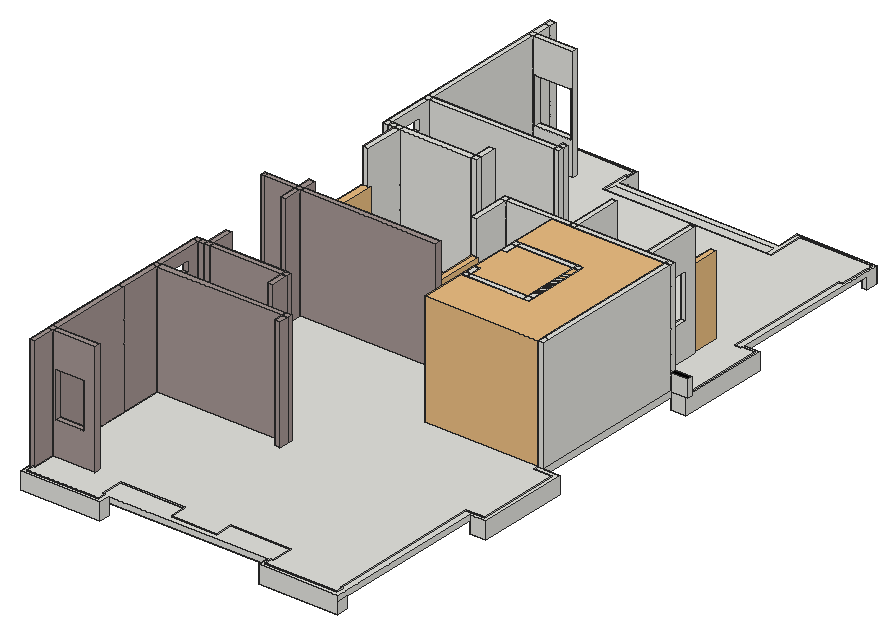
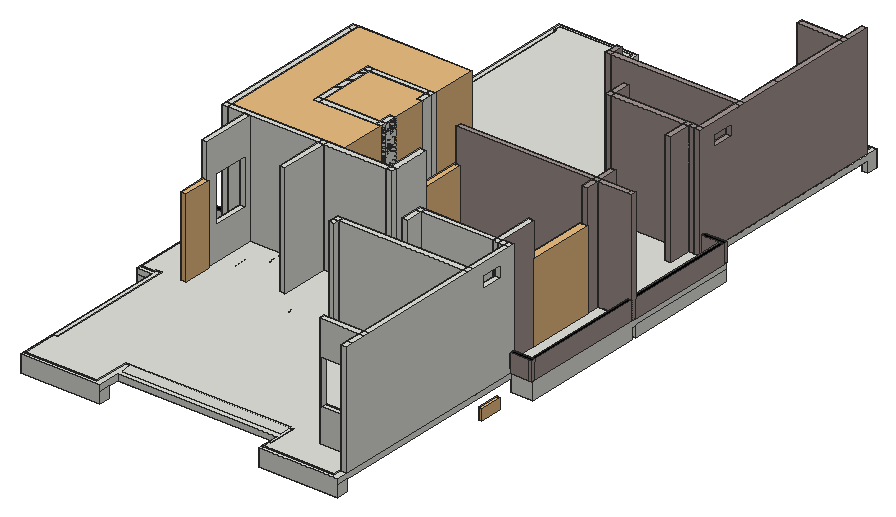
# SketchUp Ruby script. Lengths in inches.
U = 1.inch
M = Sketchup.active_model
def pt(a) = Geom::Point3d.new(a.map { |v| v * U })
def face(e, loops, mat)
  f = e.add_face(loops[0].map { |a| pt(a) })
  loops[1..].each { |l| e.add_face(l.map { |a| pt(a) }).erase! }
  f.material = f.back_material = mat if mat
  f
end
# faces: each face lists its corners as indices into pts; further lists are holes
def faces(e, pts, list, mat = nil) = list.each { |f| face(e, (f[0].is_a?(Array) ? f : [f]).map { |l| l.map { |i| pts[i] } }, mat) }
# xy, xz, yz: faces in a plane at the given z, y or x. An outline is a flat list of corners, or four numbers for a rectangle; further outlines are holes
def ring(l) = l.size == 4 ? [[l[0], l[1]], [l[2], l[1]], [l[2], l[3]], [l[0], l[3]]] : l.each_slice(2).to_a
def flat(e, list, mat, &to3) = list.each { |f| face(e, (f[0].is_a?(Array) ? f : [f]).map { |l| ring(l).map { |u, v| to3.(u, v) } }, mat) }
def xy(e, z, list, mat = nil) = flat(e, list, mat) { |x, y| [x, y, z] }
def xz(e, y, list, mat = nil) = flat(e, list, mat) { |x, z| [x, y, z] }
def yz(e, x, list, mat = nil) = flat(e, list, mat) { |y, z| [x, y, z] }
def lines(e, pts, list) = list.each { |a, b| e.add_line(pt(pts[a]), pt(pts[b])) }
# prism: a flat outline (further loops are holes) pulled along v
def prism(e, loops, v, mat = nil)
  f = face(e, loops, mat); d = Geom::Vector3d.new(v.map { |x| x * U })
  f.pushpull(f.normal.samedirection?(d) ? d.length : -d.length)
end
def box(e, o, s, mat = nil) = prism(e, [[o, [o[0] + s[0], o[1], o[2]], [o[0] + s[0], o[1] + s[1], o[2]], [o[0], o[1] + s[1], o[2]]]], [0, 0, s[2]], mat)
def at(x, y, z, deg = 0) = Geom::Transformation.translation(pt([x, y, z])) * Geom::Transformation.rotation(ORIGIN, Z_AXIS, deg.degrees)
def axes(o, x, y, z) = Geom::Transformation.new([*x, 0, *y, 0, *z, 0, *pt(o).to_a, 1])
def part(name) = M.definitions.add(name)
# library, detail: a bought-in or finely detailed component or shape, given as its bounding box
def library(name, o, s) = part(name).tap { |d| box(d.entities, o, s) }
def detail(e, o, s) = box(e.add_group.entities, o, s)
def put(e, d, t, mat = nil) = e.add_instance(d, t).tap { |i| i.material = mat if mat }
def group(e, t, mat = nil) = e.add_group.tap { |g| g.transformation = t; g.material = mat if mat }.entities
root = M.entities
M.materials.add("M09_Shadow_Night").color = [0, 0, 0]
M.materials.add("Marble_06_1K").color = [165, 150, 147]
c1 = part("Group\#53")
xy(c1.entities,0,[[-66,-66,-60,-60],[-60,-66,0,-60],[0,-66,6,-60],[-66,-60,-60,-48.73],[0,-60,6,0],
  [-66,-12.73,-60,0],[-66,0,-60,6],[-60,0,0,6],[0,0,6,6]])
xy(c1.entities,120,[[-66,-66,-60,-60],[-60,-66,0,-60],[0,-66,6,-60],[-66,-60,-60,-48.73],[0,-60,6,0],
  [-66,-12.73,-60,0],[-66,0,-60,6],[-60,0,0,6],[0,0,6,6]])
xz(c1.entities,-66,[[-66,0,-60,120],[-60,0,0,120],[0,0,6,120]])
xz(c1.entities,-60,[[-66,0,-60,120],[-60,0,0,120],[0,0,6,120]])
xz(c1.entities,-48.73,[[-66,0,-60,120]])
xz(c1.entities,-12.73,[[-66,0,-60,120]])
xz(c1.entities,0,[[-66,0,-60,120],[-60,0,0,120],[0,0,6,120]])
xz(c1.entities,6,[[-66,0,-60,120],[-60,0,0,120],[0,0,6,120]])
yz(c1.entities,-66,[[-66,0,-60,120],[-60,0,-48.73,120],[-12.73,0,0,120],[0,0,6,120]])
yz(c1.entities,-60,[[-66,0,-60,120],[-60,0,-48.73,120],[-12.73,0,0,120],[0,0,6,120]])
yz(c1.entities,0,[[-66,0,-60,120],[-60,0,0,120],[0,0,6,120]])
yz(c1.entities,6,[[-66,0,-60,120],[-60,0,0,120],[0,0,6,120]])
c2 = library("Return staircase",[0,-11.89,0],[120,168,120])
c3 = part("Group\#84")
xy(c3.entities,0,[[[-2,-32,-2,-24,0.04,-24,0.04,0,0,0,0,198,-6,198,-6,196,-25.9,196,-25.9,312.57,0,312.57,0,318.21,-25.9,318.21,-25.9,446,-6,446,-6,444,0,444,0,675.78,72,673.93,76,673.93,76,665.93,74,665.93,74,636,252.4,636,252.4,673.93,328.4,673.93,328.4,636,324.4,636,324.4,498.14,330.4,498.14,330.4,499.84,344.35,499.84,344.35,411,324.4,411,324.4,231,344.35,231,344.35,142,324.4,142,324.4,0,324.58,0,324.58,-24,326.4,-24,326.4,-32,250.4,-32,250.4,-24,252.4,-24,252.4,0,188.4,0,188.4,-18,140,-18,140,0,72,0,72,-24,74,-24,74,-32],[210.4,291,270.4,351]]])
xy(c3.entities,1,[[[-2,-32,74,-32,74,-24,72,-24,72,0,140,0,140,-18,188.4,-18,188.4,0,252.4,0,252.4,-24,250.4,-24,250.4,-32,326.4,-32,326.4,-24,324.58,-24,324.58,0,324.4,0,324.4,142,344.35,142,344.35,231,324.4,231,324.4,411,344.35,411,344.35,499.84,330.4,499.84,330.4,498.14,324.4,498.14,324.4,636,328.4,636,328.4,673.93,252.4,673.93,252.4,636,74,636,74,665.93,76,665.93,76,673.93,72,673.93,0,675.78,0,444,-6,444,-6,446,-25.9,446,-25.9,318.21,0,318.21,0,312.57,-25.9,312.57,-25.9,196,-6,196,-6,198,0,198,0,0,0.04,0,0.04,-24,-2,-24],[210.4,291,270.4,351]]])
xz(c3.entities,-32,[[-2,0,74,1],[250.4,0,326.4,1]])
xz(c3.entities,-24,[[-2,0,0.04,1],[72,0,74,1],[250.4,0,252.4,1],[324.58,0,326.4,1]])
xz(c3.entities,-18,[[140,0,188.4,1]])
xz(c3.entities,0,[[0,0,0.04,1],[72,0,140,1],[188.4,0,252.4,1],[324.4,0,324.58,1]])
xz(c3.entities,142,[[324.4,0,344.35,1]])
xz(c3.entities,196,[[-25.9,0,-6,1]])
xz(c3.entities,198,[[-6,0,0,1]])
xz(c3.entities,231,[[324.4,0,344.35,1]])
xz(c3.entities,291,[[210.4,0,270.4,1]])
xz(c3.entities,312.57,[[-25.9,0,0,1]])
xz(c3.entities,318.21,[[-25.9,0,0,1]])
xz(c3.entities,351,[[210.4,0,270.4,1]])
xz(c3.entities,411,[[324.4,0,344.35,1]])
xz(c3.entities,444,[[-6,0,0,1]])
xz(c3.entities,446,[[-25.9,0,-6,1]])
xz(c3.entities,498.14,[[324.4,0,330.4,1]])
xz(c3.entities,499.84,[[330.4,0,344.35,1]])
xz(c3.entities,636,[[74,0,252.4,1],[324.4,0,328.4,1]])
xz(c3.entities,665.93,[[74,0,76,1]])
xz(c3.entities,673.93,[[72,0,76,1],[252.4,0,328.4,1]])
yz(c3.entities,-25.9,[[196,0,312.57,1],[318.21,0,446,1]])
yz(c3.entities,-6,[[196,0,198,1],[444,0,446,1]])
yz(c3.entities,-2,[[-32,0,-24,1]])
yz(c3.entities,0,[[0,0,198,1],[312.57,0,318.21,1],[444,0,636,1],[636,0,637.85,1],[637.85,0,675.78,1]])
yz(c3.entities,0.04,[[-24,0,0,1]])
yz(c3.entities,72,[[-24,0,0,1]])
yz(c3.entities,74,[[-32,0,-24,1],[636,0,665.93,1]])
yz(c3.entities,76,[[665.93,0,673.93,1]])
yz(c3.entities,140,[[-18,0,0,1]])
yz(c3.entities,188.4,[[-18,0,0,1]])
yz(c3.entities,210.4,[[291,0,351,1]])
yz(c3.entities,250.4,[[-32,0,-24,1]])
yz(c3.entities,252.4,[[-24,0,0,1],[636,0,673.93,1]])
yz(c3.entities,270.4,[[291,0,351,1]])
yz(c3.entities,324.4,[[0,0,142,1],[231,0,411,1],[498.14,0,636,1]])
yz(c3.entities,324.58,[[-24,0,0,1]])
yz(c3.entities,326.4,[[-32,0,-24,1]])
yz(c3.entities,328.4,[[636,0,673.93,1]])
yz(c3.entities,330.4,[[498.14,0,499.84,1]])
yz(c3.entities,344.35,[[142,0,231,1],[411,0,499.84,1]])
p = [[77.67,648,0],[77.67,636,1],[246.4,636,1],[246.4,648,0],[72,673.93,0],[0,675.78,0],
  [0,675.78,1],[72,673.93,1],[70,636,0],[74,636,0],[42,642,0],[13.06,642,0],
  [13.06,673.93,0],[42,673.93,0]]
faces(c3.entities,p,[[0,1,2,3],[4,5,6,7]])
lines(c3.entities,p,[[8,9],[10,11],[12,13]])
c4 = library("TREE-26",[-60.96,-72.91,0],[121.92,134.74,0.01])
c5 = library("HYHHYHYHYHYHY",[-2.09,-4.54,0],[4.18,9.08,0.01])
c6 = library("Group\#51",[0,0,0],[6.9375,42,86.5])
c7 = part("feeeeeeeeee")
p = [[-2.68,3.51,0],[-2.68,3.16,0],[-2.92,3.16,0],[-2.92,3.07,0],[-3.56,3.07,0],[-3.56,3.51,0],
  [-2.68,-3.51,0],[-2.68,-3.16,0],[-2.92,-3.16,0],[-2.92,-3.07,0],[-3.56,-3.07,0],[-3.56,-3.51,0],
  [3.56,3.16,0],[-2.68,2.93,0],[3.56,2.93,0],[-2.48,-3.13,0],[-2.04,-3.07,0],[-1.61,-2.98,0],
  [-1.1875,-2.86,0],[-0.77,-2.72,0],[-0.36,-2.55,0],[0.03,-2.35,0],[0.41,-2.13,0],[0.78,-1.88,0],
  [1.125,-1.62,0],[1.46,-1.32,0],[1.77,-1.01,0],[2.06,-0.68,0],[2.33,-0.33,0],[2.57,0.03,0],
  [2.79,0.42,0],[2.99,0.81,0],[3.16,1.22,0],[3.3,1.63,0],[3.41,2.06,0],[3.5,2.49,0]]
lines(c7.entities,p,[[0,1],[1,2],[2,3],[3,4],[4,5],[5,0],[6,7],[7,8],[8,9],[9,10],[10,11],[11,6],
  [1,12],[13,14],[1,13],[12,14],[8,15],[15,16],[16,17],[17,18],[18,19],[19,20],[20,21],[21,22],
  [22,23],[23,24],[24,25],[25,26],[26,27],[27,28],[28,29],[29,30],[30,31],[31,32],[32,33],[33,34],
  [34,35],[35,14]])
c8 = part("Group\#12")
xy(c8.entities,0,[[0,0,6,7.18],[0,7.18,6,168],[-174.4,129.21,-168.4,168],[-174.4,168,-168.4,174],[-168.4,168,-102,174],
  [-102,168,-96,174],[-96,168,0,174],[0,168,6,174],[6,168,24,174],[-102,174,-96,225]])
xy(c8.entities,18,[[6,168,24,174]],"M09_Shadow_Night")
xy(c8.entities,120,[[0,0,6,7.18],[0,7.18,6,168],[-174.4,129.21,-168.4,168],[-174.4,168,-168.4,174],[-168.4,168,-102,174],
  [-102,168,-96,174],[-96,168,0,174],[0,168,6,174],[-102,174,-96,225]])
xz(c8.entities,0,[[0,0,6,120]])
xz(c8.entities,129.21,[[-174.4,0,-168.4,120]])
xz(c8.entities,168,[[-174.4,0,-168.4,120],[-168.4,0,-102,120],[-102,0,-96,120],[-96,0,0,120],[0,0,6,120],
  [6,0,24,18]])
xz(c8.entities,174,[[-174.4,0,-168.4,120],[-168.4,0,-102,120],[-102,0,-96,120],[-96,0,0,120],[0,0,6,120],
  [6,0,24,18]])
xz(c8.entities,225,[[-102,0,-96,120]])
yz(c8.entities,-174.4,[[129.21,0,168,120],[168,0,174,120]])
yz(c8.entities,-168.4,[[129.21,0,168,120],[168,0,174,120]])
yz(c8.entities,-102,[[168,0,174,120],[174,0,225,120]])
yz(c8.entities,-96,[[168,0,174,120],[174,0,225,120]])
yz(c8.entities,0,[[0,0,7.18,120],[7.18,0,168,120],[168,0,174,120]])
yz(c8.entities,6,[[0,0,168,120],[168,0,174,18],[168,18,174,120]])
yz(c8.entities,24,[[168,0,174,18]])
c9 = library("porta correr aluminio",[0,0,0],[4.49,110.28,83.35])
c10 = library("VVVV",[-3.39,-3.68,0],[6.78,7.36,0.01])
c11 = library("BFGFV",[-4.32,-2.51,0],[8.64,5.02,0.01])
c12 = library("Group\#115",[0,0,0],[72,16,6.2])
c13 = library("burner",[-300,-225,0],[600,450,0.01])
c14 = library("lcd-01",[-577.99,-134.75,0],[1155.98,269.5,0.01])
c15 = part("Component\#5")
p = [[1166.02,522.1,0],[1167.27,522.1,0],[1183.11,522.1,0],[1183.72,522.1,0],[1165.72,517.1,0],[1167.27,517.1,0],
  [1183.11,517.1,0],[1183.72,517.1,0],[1165.72,512.1,0],[1167.27,512.1,0],[1183.11,512.1,0],[1183.72,512.1,0],
  [1165.72,507.1,0],[1167.27,507.1,0],[1183.11,507.1,0],[1183.72,507.1,0],[1165.72,502.1,0],[1167.27,502.1,0],
  [1183.11,502.1,0],[1183.72,502.1,0],[1165.72,497.1,0],[1167.27,497.1,0],[1183.11,497.1,0],[1183.72,497.1,0],
  [1165.72,492.1,0],[1183.72,492.1,0],[1165.72,487.1,0],[1183.72,487.1,0],[1111.72,482.1,0],[1128.65,482.1,0],
  [1150.05,482.1,0],[1183.72,482.1,0],[1111.72,477.1,0],[1128.65,477.1,0],[1150.05,477.1,0],[1183.72,477.1,0],
  [1111.72,472.1,0],[1128.65,472.1,0],[1150.05,472.1,0],[1173.72,472.1,0],[1117.28,469.6,0],[1112.28,474.6,0],
  [1127.28,479.6,0],[1122.28,484.6,0],[1157.28,469.6,0],[1152.28,474.6,0],[1173.72,473.16,0],[1172.28,474.6,0],
  [1167.28,479.6,0],[1162.28,484.6,0],[1183.72,483.16,0],[1182.28,484.6,0],[1177.28,489.6,0],[1172.48,494.4,0],
  [1167.27,499.61,0],[1165.72,501.16,0],[1183.72,503.16,0],[1183.11,503.77,0],[1167.27,519.61,0],[1165.77,521.11,0],
  [1183.72,523.16,0],[1182.3,524.58,0],[1118.53,469.6,0],[1113.53,474.6,0],[1128.53,479.6,0],[1123.53,484.6,0],
  [1158.53,469.6,0],[1153.53,474.6,0],[1173.72,474.41,0],[1173.53,474.6,0],[1168.53,479.6,0],[1163.53,484.6,0],
  [1183.72,484.41,0],[1183.53,484.6,0],[1178.53,489.6,0],[1173.73,494.4,0],[1167.27,500.86,0],[1165.72,502.41,0],
  [1183.72,504.41,0],[1183.53,504.6,0],[1167.27,520.86,0],[1166.02,522.11,0],[1183.72,524.41,0],[1183.55,524.58,0],
  [1119.78,469.6,0],[1114.78,474.6,0],[1128.65,480.73,0],[1124.78,484.6,0],[1159.78,469.6,0],[1154.78,474.6,0],
  [1169.78,479.6,0],[1164.78,484.6,0],[1179.78,489.6,0],[1174.98,494.4,0],[1167.27,502.11,0],[1165.72,503.66,0],
  [1167.27,522.11,0],[1166.48,522.9,0]]
lines(c15.entities,p,[[0,1],[2,3],[4,5],[6,7],[8,9],[10,11],[12,13],[14,15],[16,17],[18,19],[20,21],[22,23],
  [24,25],[26,27],[28,29],[30,31],[32,33],[34,35],[36,37],[38,39],[40,41],[42,43],[44,45],[46,47],
  [48,49],[50,51],[52,53],[54,55],[56,57],[58,59],[60,61],[62,63],[64,65],[66,67],[68,69],[70,71],
  [72,73],[74,75],[76,77],[78,79],[80,81],[82,83],[84,85],[86,87],[88,89],[90,91],[92,93],[94,95],
  [96,97]])
c16 = library("sink",[-449.92,-250,0],[899.84,500,0.01])
c17 = library("A$C72E23588",[-1177.7,-903.95,0],[2355.4,1807.9,0.01])
c18 = library("JEEW",[-211.14,-299.86,0],[422.28,599.72,0.01])
c19 = library("ghgjg",[-265.23,-341.01,0],[530.46,682.02,0.01])
c20 = library("Group\#46",[0,-0.05,0],[30,2.55,24])
c21 = part("tgr")
p = [[-2.37,-3.35,0],[-2.37,-2.82,0],[-2.73,-2.82,0],[-2.73,-2.68,0],[-3.71,-2.68,0],[-3.71,-3.35,0],
  [-2.37,3.35,0],[-2.37,2.82,0],[-2.73,2.82,0],[-2.73,2.68,0],[-3.71,2.68,0],[-3.71,3.35,0],
  [3.71,-2.82,0],[-2.37,-2.46,0],[3.71,-2.46,0],[3.7,-2.46,0],[3.63,-2.07,0],[3.53,-1.68,0],
  [3.41,-1.3,0],[3.27,-0.93,0],[3.1,-0.57,0],[2.91,-0.22,0],[2.7,0.12,0],[2.46,0.4375,0],
  [2.21,0.74,0],[1.93,1.03,0],[1.64,1.3,0],[1.33,1.55,0],[1.01,1.79,0],[0.67,1.99,0],
  [0.32,2.18,0],[-0.04,2.35,0],[-0.41,2.49,0],[-0.8,2.6,0],[-1.18,2.69,0],[-1.58,2.76,0],
  [-1.97,2.8,0]]
lines(c21.entities,p,[[0,1],[1,2],[2,3],[3,4],[4,5],[5,0],[6,7],[7,8],[8,9],[9,10],[10,11],[11,6],
  [1,12],[13,14],[1,13],[12,14],[15,16],[16,17],[17,18],[18,19],[19,20],[20,21],[21,22],[22,23],
  [23,24],[24,25],[25,26],[26,27],[27,28],[28,29],[29,30],[30,31],[31,32],[32,33],[33,34],[34,35],
  [35,36],[36,7]])
prism(root,[[[338.2,484.34,246],[338.2,541.34,246],[338.2,541.34,366],[338.2,484.34,366]],[[338.2,490.34,282],[338.2,490.34,330],[338.2,529.34,330],[338.2,529.34,282]]],[-6,0,0])
p = [[119.8,541.34,246],[125.8,541.34,246],[37.8,391.55,246],[37.8,404.03,246],[43.8,404.03,246],[43.8,391.55,246],
  [39.25,404.03,246],[43.8,476.03,246],[43.8,517.34,246],[125.8,517.34,246],[119.8,523.34,246],[236.2,430.34,246],
  [236.2,411.61,246],[242.2,411.61,246],[242.2,424.34,246],[308.2,430.34,246],[248.2,430.34,246],[37.8,476.03,246],
  [37.8,517.34,246],[302.2,424.34,246],[302.2,364.34,246],[31.8,523.34,246],[31.8,571.34,246],[49.8,523.34,246],
  [254.2,535.34,246],[260.2,535.34,246],[317.65,541.3,246],[317.93,541.33,246],[318.2,541.34,246],[332.2,541.34,246],
  [317.12,541.19,246],[317.38,541.25,246],[236.2,478.34,246],[315.1,539.86,246],[315.28,540.07,246],[315.47,540.26,246],
  [314.65,539.18,246],[314.78,539.42,246],[314.43,538.68,246],[314.53,538.93,246],[314.28,538.15,246],[314.35,538.42,246],
  [314.93,539.64,246],[260.2,502.34,246],[314.2,502.34,246],[314.21,537.61,246],[314.24,537.88,246],[181.8,484.34,246],
  [254.2,484.34,246],[181.8,437.06,246],[181.8,437.15,246],[181.8,439.55,246],[260.2,484.34,246],[332.2,484.34,246],
  [314.2,537.34,246],[315.67,540.44,246],[315.89,540.61,246],[316.12,540.76,246],[316.36,540.89,246],[316.6,541.01,246],
  [316.86,541.11,246],[187.8,478.34,246],[187.8,439.55,246],[25.8,517.34,246],[25.8,519.34,246],[96.33,517.34,246],
  [168.92,408.27,246],[169.38,407.99,246],[174.5625,406.96,246],[175.09,407.05,246],[168.07,421.29,246],[167.68,420.92,246],
  [165.27,415.11,246],[165.29,414.57,246],[165.34,414.03,246],[165.43,413.5,246],[165.9,418.25,246],[165.71,417.75,246],
  [165.55,412.98,246],[165.9,411.96,246],[166.12,411.47,246],[171.89,407.05,246],[172.42,406.96,246],[174.03,406.91,246],
  [165.55,417.23,246],[175.62,407.17,246],[176.13,407.32,246],[176.64,407.51,246],[177.125,407.74,246],[165.43,416.71,246],
  [165.34,416.18,246],[166.66,410.54,246],[166.97,410.1,246],[177.6,407.99,246],[179.3,409.3,246],[179.67,409.6875,246],
  [166.37,411,246],[166.66,419.67,246],[166.37,419.22,246],[172.95,406.91,246],[173.49,406.89,246],[167.3125,409.6875,246],
  [167.68,409.3,246],[167.3125,420.53,246],[166.97,420.11,246],[178.06,408.27,246],[180.01,410.1,246],[166.12,418.74,246],
  [169.86,407.74,246],[170.35,407.51,246],[178.49,408.59,246],[171.36,407.17,246],[178.91,408.93,246],[165.29,415.65,246],
  [180.61,411,246],[180.86,411.47,246],[181.08,411.96,246],[170.85,407.32,246],[180.33,410.54,246],[181.27,412.47,246],
  [168.07,408.93,246],[168.49,408.59,246],[181.43,412.98,246],[181.55,413.5,246],[181.64,414.03,246],[165.71,412.47,246],
  [181.69,414.57,246],[181.71,415.11,246],[168.49,421.63,246],[96.33,530.12,246],[96.33,523.34,246],[296.2,478.34,246],
  [284.2,478.34,246],[356.2,478.34,246],[338.2,478.34,246],[49.8,517.34,246],[362.2,478.34,246],[25.8,521.34,246],
  [25.8,523.34,246],[39.25,476.03,246],[356.2,406.34,246],[356.2,418.34,246],[272.2,478.34,246],[260.2,478.34,246],
  [248.2,478.34,246],[308.2,394.34,246],[308.2,406.34,246],[308.2,478.34,246],[338.2,484.34,246],[362.2,484.34,246],
  [356.2,394.34,246],[356.2,430.34,246],[308.2,418.34,246],[39.8,414.76,246],[39.8,438,246],[41.22,467.34,246],
  [41.22,444.1,246],[41.25,438,246],[41.25,414.76,246],[37.8,427.27,246],[39.25,427.27,246],[3.8,521.34,246],
  [3.8,391.55,246],[1.8,523.34,246],[1.8,397.34,246],[39.77,467.34,246],[37.8,452.79,246],[39.25,452.79,246],
  [5.8,519.34,246],[5.8,391.55,246],[39.77,444.1,246],[180.33,419.67,246],[180.01,420.11,246],[179.67,420.53,246],
  [179.3,420.92,246],[175.09,423.17,246],[174.5625,423.26,246],[174.03,423.31,246],[175.62,423.05,246],[173.49,423.33,246],
  [181.55,416.71,246],[181.43,417.23,246],[177.6,422.23,246],[177.125,422.48,246],[172.95,423.31,246],[172.42,423.26,246],
  [181.27,417.75,246],[178.91,421.29,246],[178.49,421.63,246],[176.64,422.7,246],[181.08,418.25,246],[180.86,418.74,246],
  [181.69,415.65,246],[181.64,416.18,246],[180.61,419.22,246],[178.06,421.94,246],[176.13,422.89,246],[171.89,423.17,246],
  [171.36,423.05,246],[170.85,422.89,246],[170.35,422.7,246],[169.86,422.48,246],[169.38,422.23,246],[168.92,421.94,246]]
lines(root,p,[[0,1],[2,3],[4,5],[3,6],[7,8],[9,1],[10,0],[11,12],[13,14],[15,16],[17,18],[19,20],
  [21,22],[21,23],[24,25],[12,13],[14,19],[26,27],[27,28],[28,29],[30,31],[31,26],[11,32],[33,34],
  [34,35],[36,37],[38,39],[40,41],[41,38],[39,36],[37,42],[42,33],[43,44],[45,46],[47,48],[46,40],
  [49,50],[51,47],[52,53],[44,54],[54,45],[35,55],[55,56],[57,58],[58,59],[59,60],[60,30],[56,57],
  [61,62],[62,51],[63,64],[18,63],[52,43],[48,24],[9,65],[66,67],[68,69],[70,71],[72,73],[74,75],
  [76,77],[73,74],[75,78],[79,80],[81,82],[83,68],[77,84],[85,86],[87,88],[89,90],[91,92],[88,93],
  [94,95],[96,91],[97,98],[99,100],[100,83],[86,87],[101,102],[71,103],[103,104],[93,105],[95,106],[104,97],
  [98,107],[108,109],[92,101],[105,110],[69,85],[111,81],[110,112],[113,72],[114,115],[115,116],[117,111],[118,114],
  [116,119],[120,121],[82,99],[122,123],[109,117],[112,94],[123,124],[67,108],[106,118],[125,79],[119,122],[124,126],
  [126,127],[84,89],[90,113],[128,70],[102,120],[107,76],[78,125],[80,96],[121,66],[129,130],[131,132],[133,134],
  [23,130],[23,135],[136,133],[6,4],[137,138],[64,137],[65,135],[135,8],[139,17],[130,65],[43,25],[130,10],
  [140,141],[132,142],[143,144],[145,146],[147,131],[134,147],[148,149],[150,140],[142,143],[144,32],[32,61],[151,133],
  [141,151],[146,152],[152,15],[134,148],[153,154],[155,156],[7,139],[157,158],[3,159],[159,160],[161,162],[138,163],
  [137,161],[163,164],[154,157],[158,153],[165,155],[166,17],[160,6],[139,167],[168,169],[167,166],[64,168],[156,170],
  [170,165],[171,172],[173,174],[175,176],[176,177],[178,175],[177,179],[180,181],[182,183],[179,184],[184,185],[181,186],
  [172,173],[187,188],[183,189],[190,191],[192,193],[186,190],[191,194],[174,187],[194,171],[127,192],[188,195],[189,196],
  [196,178],[185,197],[198,199],[200,201],[201,202],[202,203],[203,128],[197,198],[195,182],[199,200],[193,180],[16,11],
  [16,144]])
g1 = group(root,at(25.8,731.54,246))
xy(g1,0,[[12,-255.51,18,-214.2],[0,-214.2,6,-208.2],[6,-214.2,12,-208.2],[12,-214.2,18,-208.2],[18,-214.2,94,-208.2],
  [94,-214.2,100,-208.2],[0,-208.2,6,-160.2],[94,-208.2,100,-190.2],[0,-160.2,6,-154.2],[6,-160.2,138,-154.2],
  [138,-160.2,144,-154.2],[0,-154.2,6,-116.77],[138,-154.2,144,-148.2],[0,-116.77,6,-80.17],[0,-80.17,6,-22.2],
  [0,-22.2,6,-16.2],[6,-22.2,48,-16.2],[0,-16.2,6,0],[0,0,6,7.73]])
xy(g1,36,[[8,-22.2,46,-16.2]])
xy(g1,84,[[8,-22.2,46,-16.2]])
xy(g1,96,[[0,-196.2,6,-172.2]])
xy(g1,108,[[0,-196.2,6,-172.2]])
xy(g1,120,[[12,-255.51,18,-214.2],[0,-214.2,6,-208.2],[6,-214.2,12,-208.2],[12,-214.2,18,-208.2],[18,-214.2,94,-208.2],
  [94,-214.2,100,-208.2],[0,-208.2,6,-160.2],[94,-208.2,100,-190.2],[0,-160.2,6,-154.2],[6,-160.2,138,-154.2],
  [138,-160.2,144,-154.2],[0,-154.2,6,-22.2],[138,-154.2,144,-148.2],[0,-22.2,6,-16.2],[6,-22.2,48,-16.2],
  [0,-16.2,6,0],[0,0,6,7.73]])
xz(g1,-255.51,[[12,0,18,120]])
xz(g1,-214.2,[[0,0,6,120],[6,0,12,120],[12,0,18,120],[18,0,94,120],[94,0,100,120]])
xz(g1,-208.2,[[6,0,12,120],[12,0,18,120],[18,0,94,120],[94,0,100,120]])
xz(g1,-196.2,[[0,96,6,108]])
xz(g1,-190.2,[[94,0,100,120]])
xz(g1,-172.2,[[0,96,6,108]])
xz(g1,-160.2,[[6,0,138,120],[138,0,144,120]])
xz(g1,-154.2,[[6,0,138,120],[138,0,144,120]])
xz(g1,-148.2,[[138,0,144,120]])
xz(g1,-22.2,[[[6,0,48,120],[8,36,46,84]]])
xz(g1,-16.2,[[[6,0,48,120],[8,36,46,84]]])
xz(g1,7.73,[[0,0,6,120]])
yz(g1,0,[[[-214.2,0,7.73,120],[-196.2,96,-172.2,108]]])
yz(g1,6,[[-214.2,0,-208.2,120],[[-208.2,0,-160.2,120],[-196.2,96,-172.2,108]],[-160.2,0,-154.2,120],[-154.2,0,-22.2,120],[-22.2,0,-16.2,120],
  [-16.2,0,0,120],[0,0,7.73,120]])
yz(g1,8,[[-22.2,36,-16.2,84]])
yz(g1,12,[[-214.2,0,-208.2,120]])
yz(g1,12,[[-255.51,0,-214.2,120]],"Marble_06_1K")
yz(g1,18,[[-255.51,0,-214.2,120],[-214.2,0,-208.2,120]])
yz(g1,46,[[-22.2,36,-16.2,84]])
yz(g1,48,[[-22.2,0,-16.2,120]])
yz(g1,94,[[-214.2,0,-208.2,120],[-208.2,0,-190.2,120]])
yz(g1,100,[[-214.2,0,-208.2,120],[-208.2,0,-190.2,120]])
yz(g1,138,[[-160.2,0,-154.2,120],[-154.2,0,-148.2,120]])
yz(g1,144,[[-160.2,0,-154.2,120],[-154.2,0,-148.2,120]])
g2 = group(g1,at(-2.625,-212.2,0),"Marble_06_1K")
xy(g2,0,[[2.625,-470,8.625,-446],[2.625,-446,8.625,-440],[8.625,-446,53.03,-440],[2.625,-440,8.625,-352.75],[2.625,-352.75,8.625,-308],
  [140.625,-317.47,146.625,-308],[2.625,-308,8.625,-302],[8.625,-308,140.625,-302],[140.625,-308,146.625,-302],[2.625,-302,8.625,-254],
  [96.625,-272,102.625,-254],[-21.375,-254,-17.27,-250],[-17.27,-254,2.625,-250],[2.625,-254,8.625,-250],[8.625,-254,14.625,-250],
  [14.625,-254,20.625,-250],[20.625,-254,96.625,-250],[96.625,-254,102.625,-250],[-21.375,-250,-17.27,-133.43],[2.625,-250,8.625,-248],
  [8.625,-250,14.625,-248],[14.625,-250,20.625,-248],[20.625,-250,96.625,-248],[96.625,-250,102.625,-248],[14.625,-248,20.625,-224],
  [14.625,-152,20.625,-133.43],[-21.375,-133.43,-17.27,-127.79],[-17.27,-133.43,14.625,-127.79],[14.625,-133.43,20.625,-127.79],[20.625,-133.43,164.625,-127.79],
  [-21.375,-127.79,-17.27,0],[14.625,-127.79,20.625,-114.45],[-21.375,0,-17.27,4],[-17.27,0,2.625,4]])
xy(g2,20,[[-21.375,-254,2.625,-250],[-21.375,-250,-17.27,-133.43],[-21.375,-127.79,-17.27,0],[-21.375,0,2.625,4]],"M09_Shadow_Night")
xy(g2,36,[[11.33,-446,41.03,-440]])
xy(g2,84,[[11.33,-446,41.03,-440]])
xy(g2,96,[[2.625,-290,8.625,-266]])
xy(g2,108,[[2.625,-290,8.625,-266]])
xy(g2,119.9375,[[96.625,-272,102.625,-254]])
xy(g2,120,[[2.625,-470,8.625,-446],[2.625,-446,8.625,-440],[8.625,-446,53.03,-440],[2.625,-440,8.625,-352.75],[2.625,-352.75,8.625,-308],
  [140.625,-317.47,146.625,-308],[2.625,-308,8.625,-302],[8.625,-308,140.625,-302],[140.625,-308,146.625,-302],[2.625,-302,8.625,-254],
  [2.625,-254,8.625,-248],[8.625,-254,14.625,-248],[14.625,-254,20.625,-248],[20.625,-254,96.625,-248],[96.625,-254,102.625,-248],
  [14.625,-248,20.625,-224],[14.625,-152,20.625,-133.43],[-21.375,-133.43,-17.27,-127.79],[-17.27,-133.43,14.625,-127.79],[14.625,-133.43,20.625,-127.79],
  [20.625,-133.43,164.625,-127.79],[14.625,-127.79,20.625,-114.45]])
xz(g2,-470,[[2.625,0,8.625,120]])
xz(g2,-446,[[[8.625,0,53.03,120],[11.33,36,41.03,84]]],"Marble_06_1K")
xz(g2,-440,[[[8.625,0,53.03,120],[11.33,36,41.03,84]]])
xz(g2,-317.47,[[140.625,0,146.625,120]])
xz(g2,-308,[[8.625,0,140.625,120],[140.625,0,146.625,120]])
xz(g2,-302,[[8.625,0,140.625,120],[140.625,0,146.625,120]])
xz(g2,-290,[[2.625,96,8.625,108]])
xz(g2,-272,[[96.625,0,102.625,119.9375]])
xz(g2,-266,[[2.625,96,8.625,108]])
xz(g2,-254,[[-21.375,0,-17.27,20],[-17.27,0,2.625,20],[8.625,0,14.625,120],[14.625,0,20.625,120],[20.625,0,96.625,120],
  [96.625,0,102.625,119.9375],[96.625,119.9375,102.625,120]])
xz(g2,-250,[[-21.375,0,-17.27,20],[-17.27,0,2.625,20]])
xz(g2,-248,[[2.625,0,8.625,120],[8.625,0,14.625,120],[14.625,0,20.625,120],[20.625,0,96.625,120],[96.625,0,102.625,120]])
xz(g2,-224,[[14.625,0,20.625,120]])
xz(g2,-152,[[14.625,0,20.625,120]])
xz(g2,-133.43,[[-21.375,0,-17.27,20],[-17.27,0,14.625,120],[14.625,0,20.625,120],[20.625,0,164.625,120],[-21.375,20,-17.27,120]])
xz(g2,-127.79,[[-17.27,0,-17.27,20,-21.375,20,-21.375,120,14.625,120,14.625,0],[-21.375,0,-17.27,20],[14.625,0,20.625,120],[20.625,0,164.625,120]])
xz(g2,-114.45,[[14.625,0,20.625,120]])
xz(g2,0,[[-21.375,0,-17.27,20],[-17.27,0,2.625,20]])
xz(g2,4,[[-21.375,0,-17.27,20],[-17.27,0,2.625,20]])
yz(g2,-21.375,[[-254,0,-250,20],[-250,0,-133.43,20],[-133.43,0,-127.79,120],[-127.79,0,0,20],[0,0,4,20]])
yz(g2,-17.27,[[-250,0,-133.43,20],[-127.79,0,0,20]])
yz(g2,2.625,[[[-470,0,-470,120,-248,120,-248,0,-250,0,-250,20,-254,20,-254,0],[-290,96,-266,108]],[-254,0,-250,20],[0,0,4,20]])
yz(g2,8.625,[[-446,0,-440,120],[-440,0,-352.75,120],[-352.75,0,-308,120],[-308,0,-302,120],[[-302,0,-254,120],[-290,96,-266,108]],
  [-254,0,-248,120]])
yz(g2,8.625,[[-470,0,-446,120]],"Marble_06_1K")
yz(g2,11.33,[[-446,36,-440,84]])
yz(g2,14.625,[[-254,0,-248,120],[-248,0,-224,120],[-152,0,-133.43,120],[-133.43,0,-127.79,120],[-127.79,0,-114.45,120]])
yz(g2,20.625,[[-254,0,-248,120],[-248,0,-224,120],[-152,0,-133.43,120],[-133.43,0,-127.79,120],[-127.79,0,-114.45,120]])
yz(g2,41.03,[[-446,36,-440,84]])
yz(g2,53.03,[[-446,0,-440,120]])
yz(g2,96.625,[[-272,0,-254,119.9375],[-254,0,-248,120]])
yz(g2,102.625,[[-272,0,-254,119.9375],[-254,0,-248,120]])
yz(g2,140.625,[[-317.47,0,-308,120],[-308,0,-302,120]])
yz(g2,146.625,[[-317.47,0,-308,120],[-308,0,-302,120]])
yz(g2,164.625,[[-133.43,0,-127.79,120]])
g3 = group(root,at(25.8,49.34,264.53))
xy(g3,-36.67,[[252.4,-12,252.4,0,259.49,0,259.49,-8,330.4,-8,330.4,0,336.4,0,336.4,-12]])
xy(g3,-36.53,[[0,-12,0,-0.08,6,-0.08,6,-8,78,-8,78,0,84,0,84,-12],[336.4,163,336.4,169,349.41,169,349.41,255,336.4,255,336.4,261,353.41,261,353.41,163],[-24,217,-24,336.57,-20,336.57,-20,222,0,222,0,217],[-24,342.21,-24,473,0,473,0,468,-20,468,-20,342.21],[336.4,430,336.4,435,347.875,435,347.875,523,335.62,523,335.62,528,351.875,528,351.875,430],
  [0,689.93,0,701.93,84,701.93,84,689.93,78,689.93,78,697.93,6,697.93,6,689.93],[252.4,689.93,252.4,701.93,336.4,701.93,336.4,689.93,330.4,689.93,330.4,697.93,258.4,697.93,258.4,689.93]])
xy(g3,-24.53,[[[6,-8,6,-0.08,0,-0.08,0,222,-20,222,-20,336.57,-24,336.57,-24,342.21,-20,342.21,-20,468,0,468,0,689.93,6,689.93,6,697.93,78,697.93,78,689.93,84,689.93,84,678,252.4,678,252.4,689.93,258.4,689.93,258.4,697.93,330.4,697.93,330.4,689.93,336.4,689.93,336.4,528,335.62,528,335.62,523,347.875,523,347.875,435,336.4,435,336.4,255,349.41,255,349.41,169,336.4,169,336.4,0,330.4,0,330.4,-8,259.49,-8,259.49,0,78,0,78,-8],[216.4,315,276.4,375]],[-24,217,0,217,0,222,-20,222,-20,336.57,-24,336.57]])
xy(g3,-18.53,[[[0,-12,84,-12,84,0,252.4,0,252.4,-12,336.4,-12,336.4,163,353.41,163,353.41,261,336.4,261,336.4,430,351.875,430,351.875,528,336.4,528,336.4,701.93,252.4,701.93,252.4,678,84,678,84,701.93,0,701.93,0,473,-24,473,-24,217,0,217],[216.4,315,276.4,375]]])
xz(g3,-12,[[252.4,-36.67,336.4,-18.53],[0,-36.53,84,-18.53]])
xz(g3,-8,[[259.49,-36.67,330.4,-24.53],[6,-36.53,78,-24.53]])
xz(g3,-0.08,[[0,-36.53,6,-24.53]])
xz(g3,0,[[252.4,-36.67,259.49,-24.53],[330.4,-36.67,336.4,-24.53],[78,-36.53,84,-24.53],[84,-24.53,252.4,-18.53]])
xz(g3,163,[[336.4,-36.53,353.41,-18.53]])
xz(g3,169,[[336.4,-36.53,349.41,-24.53]])
xz(g3,217,[[-24,-36.53,0,-24.53],[-24,-24.53,0,-18.53]])
xz(g3,222,[[-20,-36.53,0,-24.53]])
xz(g3,255,[[336.4,-36.53,349.41,-24.53]])
xz(g3,261,[[336.4,-36.53,353.41,-18.53]])
xz(g3,315,[[216.4,-24.53,276.4,-18.53]])
xz(g3,336.57,[[-24,-36.53,-20,-24.53]])
xz(g3,342.21,[[-24,-36.53,-20,-24.53]])
xz(g3,375,[[216.4,-24.53,276.4,-18.53]])
xz(g3,430,[[336.4,-36.53,351.875,-18.53]])
xz(g3,435,[[336.4,-36.53,347.875,-24.53]])
xz(g3,468,[[-20,-36.53,0,-24.53]])
xz(g3,473,[[-24,-36.53,0,-18.53]])
xz(g3,523,[[335.62,-36.53,347.875,-24.53]])
xz(g3,528,[[335.62,-36.53,351.875,-24.53],[336.4,-24.53,351.875,-18.53]])
xz(g3,678,[[84,-24.53,252.4,-18.53]])
xz(g3,689.93,[[0,-36.53,6,-24.53],[78,-36.53,84,-24.53],[252.4,-36.53,258.4,-24.53],[330.4,-36.53,336.4,-24.53]])
xz(g3,697.93,[[6,-36.53,78,-24.53],[258.4,-36.53,330.4,-24.53]])
xz(g3,701.93,[[0,-36.53,84,-18.53],[252.4,-36.53,336.4,-18.53]])
yz(g3,-24,[[217,-36.53,336.57,-24.53],[342.21,-36.53,342.21,-24.53,217,-24.53,217,-18.53,473,-18.53,473,-36.53]])
yz(g3,-20,[[222,-36.53,336.57,-24.53],[342.21,-36.53,468,-24.53]])
yz(g3,0,[[-12,-36.53,-12,-18.53,217,-18.53,217,-24.53,-0.08,-24.53,-0.08,-36.53],[217,-36.53,222,-24.53],[468,-36.53,473,-24.53],[689.93,-36.53,701.93,-24.53],[473,-24.53,701.93,-18.53]])
yz(g3,6,[[-8,-36.53,-0.08,-24.53],[689.93,-36.53,697.93,-24.53]])
yz(g3,78,[[-8,-36.53,0,-24.53],[689.93,-36.53,697.93,-24.53]])
yz(g3,84,[[-12,-36.53,0,-18.53],[689.93,-36.53,701.93,-36.53,701.93,-18.53,678,-18.53,678,-24.53,689.93,-24.53]])
yz(g3,216.4,[[315,-24.53,375,-18.53]])
yz(g3,252.4,[[-12,-36.67,0,-18.53],[689.93,-36.53,701.93,-24.53],[678,-24.53,701.93,-18.53]])
yz(g3,258.4,[[689.93,-36.53,697.93,-24.53]])
yz(g3,259.49,[[-8,-36.67,0,-24.53]])
yz(g3,276.4,[[315,-24.53,375,-18.53]])
yz(g3,330.4,[[-8,-36.67,0,-24.53],[689.93,-36.53,697.93,-24.53]])
yz(g3,335.62,[[523,-36.53,528,-24.53]])
yz(g3,336.4,[[-12,-36.67,0,-24.53],[163,-36.53,169,-24.53],[255,-36.53,261,-24.53],[430,-36.53,435,-24.53],[689.93,-36.53,701.93,-36.53,701.93,-18.53,528,-18.53,528,-24.53,689.93,-24.53],
  [-12,-24.53,163,-18.53],[261,-24.53,430,-18.53]])
yz(g3,347.875,[[435,-36.53,523,-24.53]])
yz(g3,349.41,[[169,-36.53,255,-24.53]])
yz(g3,351.875,[[430,-36.53,528,-18.53]])
yz(g3,353.41,[[163,-36.53,261,-18.53]])
put(root,c1,at(302.2,424.34,246))
put(root,c2,at(236.2,322.23,246))
put(root,c3,at(31.8,73.34,246))
put(root,c4,axes([12.58,398.13,246],[0,0.1317,0],[0.1317,0,0],[0,0,0.1317]))
put(root,c5,axes([99.08,410.24,246],[0,-6.75189,0],[6.75189,0,0],[0,0,6.75189]))
put(root,c6,axes([189.46,439.01,246],[-0.85622,0,0],[0,-1.13,0],[0,0,0.9711]))
put(root,c7,axes([163.46,415.55,246],[-6.83664,0,0],[0,-6.83664,0],[0,0,6.83664]))
put(root,c8,at(356.2,310.34,246))
put(root,c9,axes([45.93,404.95,246.65],[-1.89519,0,0],[0,0.65291,0],[0,0,1]))
put(root,c10,axes([64.42,443.33,246],[4.47564,0,0],[0,4.47564,0],[0,0,4.47564]))
put(root,c10,axes([138,443.33,246],[-4.47564,0,0],[0,4.47564,0],[0,0,4.47564]))
put(root,c11,axes([101.4,444.26,246],[4.3395,0,0],[0,4.3395,0],[0,0,4.3395]))
put(root,c12,axes([5.8,506.12,234.2],[0,-1.5912,0],[2,0,0],[0,0,-1]))
put(root,c13,axes([287.83,493.58,246],[-0.03566,0,0],[0,-0.03566,0],[0,0,0.03566]))
put(root,c14,axes([102.68,511.95,246],[0.04,0,0],[0,0.04,0],[0,0,0.04]))
put(root,c15,at(-851.52,16.76,246))
put(root,c4,axes([12.58,513.99,246],[0,0.1317,0],[0.1317,0,0],[0,0,0.1317]))
put(root,c16,axes([323.67,525.41,246],[0,0.03168,0],[0.03168,0,0],[0,0,0.03168]))
put(root,c17,axes([191.83,525.47,246],[0.0356,0,0],[0,-0.0356,0],[0,0,0.0356]))
put(root,c18,axes([106.95,532.38,246],[0,-0.04284,0],[-0.04284,0,0],[0,0,0.04284]))
put(root,c19,axes([45.4375,547.34,246],[0,-0.04,0],[-0.04,0,0],[0,0,0.04]))
put(root,c20,axes([26.6,559.34,216],[0,-0.8,0],[1.27878,0,0],[0,0,0.5]))
put(root,c21,axes([348.8,556.34,246],[4.47464,0,0],[0,-4.47464,0],[0,0,4.47464]))
put(root,c6,axes([330.54,541.34,246],[0.85622,0,0],[0,0.71429,0],[0,0,0.9711]))
put(root,c21,axes([109.2,556.34,246],[-4.47464,0,0],[0,-4.47464,0],[0,0,4.47464]))
